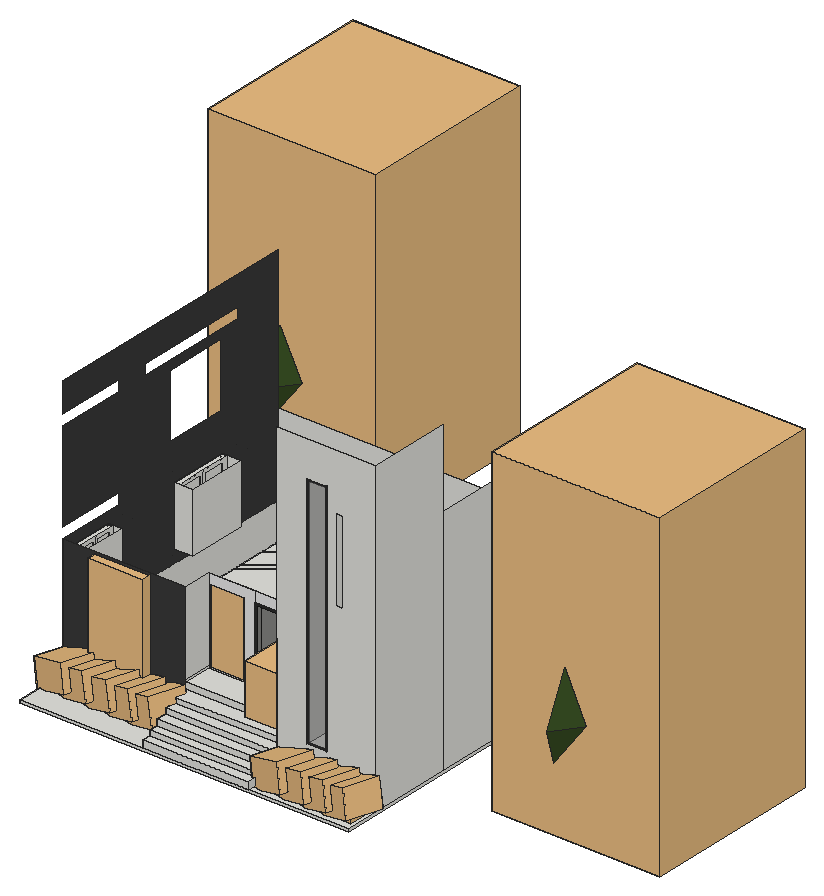
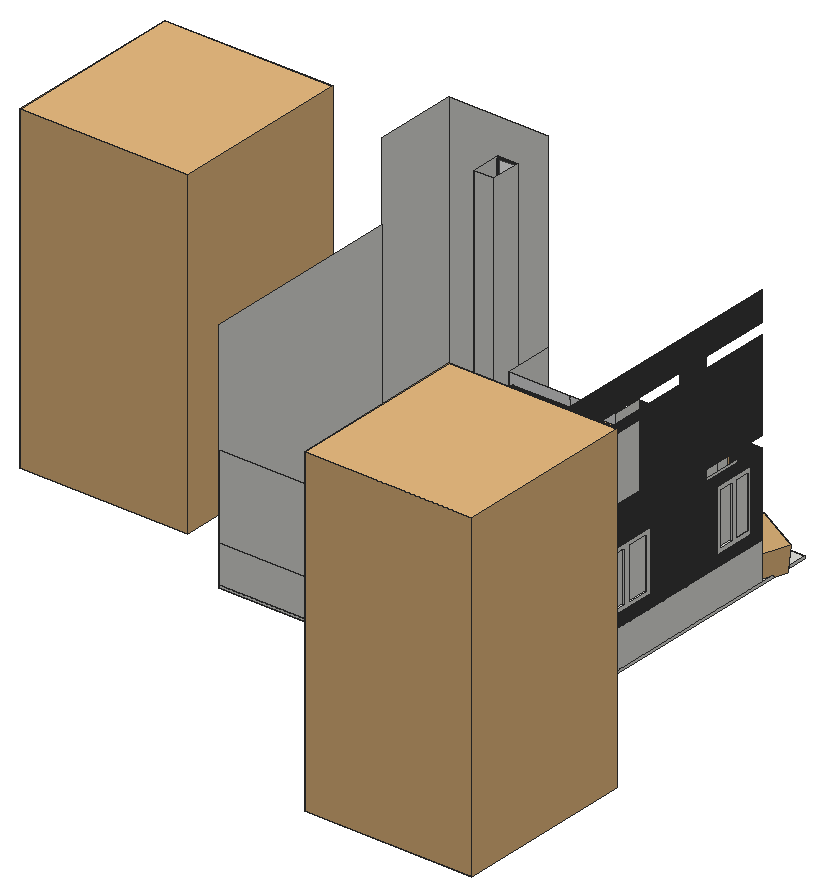
# SketchUp Ruby script. Lengths in inches.
U = 1.inch
M = Sketchup.active_model
def pt(a) = Geom::Point3d.new(a.map { |v| v * U })
def face(e, loops, mat)
  f = e.add_face(loops[0].map { |a| pt(a) })
  loops[1..].each { |l| e.add_face(l.map { |a| pt(a) }).erase! }
  f.material = f.back_material = mat if mat
  f
end
# faces: each face lists its corners as indices into pts; further lists are holes
def faces(e, pts, list, mat = nil) = list.each { |f| face(e, (f[0].is_a?(Array) ? f : [f]).map { |l| l.map { |i| pts[i] } }, mat) }
# xy, xz, yz: faces in a plane at the given z, y or x. An outline is a flat list of corners, or four numbers for a rectangle; further outlines are holes
def ring(l) = l.size == 4 ? [[l[0], l[1]], [l[2], l[1]], [l[2], l[3]], [l[0], l[3]]] : l.each_slice(2).to_a
def flat(e, list, mat, &to3) = list.each { |f| face(e, (f[0].is_a?(Array) ? f : [f]).map { |l| ring(l).map { |u, v| to3.(u, v) } }, mat) }
def xy(e, z, list, mat = nil) = flat(e, list, mat) { |x, y| [x, y, z] }
def xz(e, y, list, mat = nil) = flat(e, list, mat) { |x, z| [x, y, z] }
def yz(e, x, list, mat = nil) = flat(e, list, mat) { |y, z| [x, y, z] }
def lines(e, pts, list) = list.each { |a, b| e.add_line(pt(pts[a]), pt(pts[b])) }
# prism: a flat outline (further loops are holes) pulled along v
def prism(e, loops, v, mat = nil)
  f = face(e, loops, mat); d = Geom::Vector3d.new(v.map { |x| x * U })
  f.pushpull(f.normal.samedirection?(d) ? d.length : -d.length)
end
def box(e, o, s, mat = nil) = prism(e, [[o, [o[0] + s[0], o[1], o[2]], [o[0] + s[0], o[1] + s[1], o[2]], [o[0], o[1] + s[1], o[2]]]], [0, 0, s[2]], mat)
def at(x, y, z, deg = 0) = Geom::Transformation.translation(pt([x, y, z])) * Geom::Transformation.rotation(ORIGIN, Z_AXIS, deg.degrees)
def axes(o, x, y, z) = Geom::Transformation.new([*x, 0, *y, 0, *z, 0, *pt(o).to_a, 1])
def part(name) = M.definitions.add(name)
# library, detail: a bought-in or finely detailed component or shape, given as its bounding box
def library(name, o, s) = part(name).tap { |d| box(d.entities, o, s) }
def detail(e, o, s) = box(e.add_group.entities, o, s)
def put(e, d, t, mat = nil) = e.add_instance(d, t).tap { |i| i.material = mat if mat }
def group(e, t, mat = nil) = e.add_group.tap { |g| g.transformation = t; g.material = mat if mat }.entities
root = M.entities
M.materials.add("AM113_062_Tilia").color = [58, 81, 37]
M.materials.add("AM113_062_Tilia_Bark").color = [88, 85, 72]
M.materials.add("Glass_Tinted_Gray").color = [0, 0, 0]
M.materials["Glass_Tinted_Gray"].alpha = 0.125
M.materials.add("Material__1").color = [190, 136, 85]
M.materials.add("Material__2").color = [51, 42, 44]
M.materials.add("Material__3").color = [119, 136, 107]
M.materials.add("[0135_DarkGray]").color = [81, 81, 81]
M.materials.add("[Color M07]").color = [58, 58, 58]
M.materials.add("[Mirror 02]").color = [229, 229, 229]
M.materials.add("[Terrazzo Light Blue]").color = [196, 214, 227]
M.materials.add("[Translucent Glass Gray]1").color = [128, 128, 128]
M.materials["[Translucent Glass Gray]1"].alpha = 0.5
M.materials.add("white_wall").color = [233, 233, 233]
c1 = library("\#2",[-119.83,-119.83,113.8],[239.66,239.66,17.4])
c2 = library("\#4",[-204.92,-212.35,-236.71],[424.28,257.5,472.53])
c3 = part("\#3")
put(c3.entities,c2,axes([-0.37,309.72,0],[1.36765,0,0],[0,1.36765,0],[0,0,1.36765]),"Material__3")
c4 = library("\#1",[-174.07,-174.07,0],[348.14,348.14,140])
c5 = part("9")
put(c5.entities,c1,at(-19.94,-24.66,0),"Material__2")
put(c5.entities,c3,axes([17.67,-32.6,40.29],[0.29694,0.9549,0],[-0.21403,0.06656,0.97456],[0.9306,-0.28939,0.22414]))
put(c5.entities,c4,at(-19.94,-24.66,0),"Material__1")
c6 = library("AM113_062_Tilia_Defintion",[-350.67,-364.73,-2.58],[672.29,726.36,1000])
c7 = library("Shrub+_Grass",[-121.83,-22.34,0],[123.96,19.94,123.95])
c8 = library("Plant",[-21.8,-11.875,0],[94.69,106.42,111.78])
c9 = library("PINTU+6+YA",[0,-0.6875,0],[35.83,8.07,80.71])
c10 = part("PENTEK_RP Fineline 50S_Sliding_DoorCase_E1")
box(c10.entities,[0,0,0],[1.51,3.66,99.27],"[0135_DarkGray]")
c11 = part("PENTEK_RP Fineline 50S_SlidingDooe_Case_E2")
box(c11.entities,[0,0,0],[96.25,3.66,1.51],"[0135_DarkGray]")
c12 = part("pentek_RP Fineline 50S_SlidingDoor_Case")
put(c12.entities,c10,at(97.76,0,0))
put(c12.entities,c11,at(1.51,0,0))
put(c12.entities,c10,at(0,0,0))
put(c12.entities,c11,at(1.51,0,97.76))
c13 = part("PENTEK_RP Fineline 50S_SlidingDoor_GlazingBead_2")
box(c13.entities,[0,0,0],[0.56,0.59,94.39],"[0135_DarkGray]")
c14 = part("PENTEK_RP Fineline 50S_SlidingDoor_Glass")
box(c14.entities,[0,0,0],[46.58,0.16,94.39],"Glass_Tinted_Gray")
c15 = part("PENTEK_RP Fineline 50S_SlidingDoor_GlazingBead")
box(c15.entities,[0,0,0],[45.47,0.59,0.56],"[0135_DarkGray]")
c16 = part("PENTEK_RP Fineline 50S_SlidingDoor_Leaf_E1")
xy(c16.entities,0,[[0,0,0.93,1.97],[0.93,1.57,1.49,1.97]],"[0135_DarkGray]")
xy(c16.entities,96.25,[[0,0,0.93,0,0.93,1.57,1.49,1.57,1.49,1.97,0,1.97]],"[0135_DarkGray]")
xz(c16.entities,0,[[0,0,0.93,96.25]],"[0135_DarkGray]")
xz(c16.entities,1.57,[[0.93,0,1.49,95.32],[0.93,95.32,1.49,96.25]],"[0135_DarkGray]")
xz(c16.entities,1.97,[[0,0,1.49,96.25]],"[0135_DarkGray]")
yz(c16.entities,0,[[0,0,1.97,96.25]],"[0135_DarkGray]")
yz(c16.entities,0.93,[[0,0,1.57,0.93],[0,0.93,1.57,95.32],[0,95.32,1.57,96.25]],"[0135_DarkGray]")
yz(c16.entities,1.49,[[1.57,0,1.97,95.32],[1.57,95.32,1.97,96.25]],"[0135_DarkGray]")
c17 = part("PENTEK_RP Fineline 50S_SlidingDoor_Leaf_E2")
xy(c17.entities,0,[[0,0,0,1.57,0.56,1.57,0.56,1.97,46.02,1.97,46.02,1.57,46.58,1.57,46.58,0]],"[0135_DarkGray]")
xy(c17.entities,0.93,[[0,0,46.58,1.57]],"[0135_DarkGray]")
xy(c17.entities,1.49,[[0.56,1.57,46.02,1.97]],"[0135_DarkGray]")
xz(c17.entities,0,[[0,0,46.58,0.93]],"[0135_DarkGray]")
xz(c17.entities,1.57,[[0,0,0.56,0.93],[46.02,0,46.58,0.93],[0.56,0.93,46.02,1.49]],"[0135_DarkGray]")
xz(c17.entities,1.97,[[0.56,0,46.02,1.49]],"[0135_DarkGray]")
yz(c17.entities,0,[[0,0,1.57,0.93]],"[0135_DarkGray]")
yz(c17.entities,0.56,[[1.57,0,1.97,0.93],[1.57,0.93,1.97,1.49]],"[0135_DarkGray]")
yz(c17.entities,46.02,[[1.57,0,1.97,0.93],[1.57,0.93,1.97,1.49]],"[0135_DarkGray]")
yz(c17.entities,46.58,[[0,0,1.57,0.93]],"[0135_DarkGray]")
c18 = part("PENTEK_RP Fineline S_SlidingDoor_Leaf1")
put(c18.entities,c13,at(0.93,0,0.93))
put(c18.entities,c13,at(46.96,0,0.93))
put(c18.entities,c14,at(1.49,1.42,0.93))
put(c18.entities,c15,at(1.49,0,0.93))
put(c18.entities,c14,at(1.49,0.59,0.93),"[Terrazzo Light Blue]")
put(c18.entities,c16,at(0,0,0))
put(c18.entities,c16,axes([48.44,0,0],[-1,0,0],[0,1,0],[0,0,1]))
put(c18.entities,c17,axes([0.93,0,96.25],[1,0,0],[0,1,0],[0,0,-1]))
put(c18.entities,c17,at(0.93,0,0))
put(c18.entities,c15,at(1.49,0,94.77))
c19 = part("PENTEK_RP Fineline 50S_SlidingDoor_Leaf2")
put(c19.entities,c14,at(1.49,1.42,0.93))
put(c19.entities,c15,at(1.49,0,94.77))
put(c19.entities,c13,at(46.96,0,0.93))
put(c19.entities,c14,at(1.49,0.59,0.93),"[Mirror 02]")
put(c19.entities,c13,at(0.93,0,0.93))
put(c19.entities,c16,at(0,0,0))
put(c19.entities,c16,axes([48.44,0,0],[-1,0,0],[0,1,0],[0,0,1]))
put(c19.entities,c15,at(1.49,0,0.93))
put(c19.entities,c17,axes([0.93,0,96.25],[1,0,0],[0,1,0],[0,0,-1]))
put(c19.entities,c17,at(0.93,0,0))
c20 = part("PENTEK - Slimmest Steel Sliding Door / Window\#1")
put(c20.entities,c12,at(0,-1.88,-0.09))
put(c20.entities,c18,at(1.51,-2.27,1.42))
put(c20.entities,c19,at(49.32,-0.3,1.42))
c21 = part("Window (2)")
xy(c21.entities,31.72,[[-0.78,88.6,2.72,128.1]])
xy(c21.entities,34.95,[[-0.78,91.53,0.84,106.59],[0.84,91.53,1.05,97.58],[1.05,91.53,1.42,106.59],[1.42,91.53,2.72,106.59],[0.84,97.58,1.05,98.18],
  [0.84,98.18,1.05,106.59]])
xy(c21.entities,35.27,[[-0.78,110.09,0.97,125.14],[1.05,110.09,2.72,125.14]])
xy(c21.entities,58.35,[[2.72,108.74,3.8,109.74]])
xy(c21.entities,77.8125,[[-0.78,110.09,2.72,125.14],[0.97,110.09,1.05,125.14]])
xy(c21.entities,77.93,[[-0.78,91.53,0.84,106.59],[1.05,91.53,1.42,106.59],[1.42,91.53,2.72,106.59]])
xy(c21.entities,80.72,[[-0.78,88.6,2.72,128.1]])
xz(c21.entities,88.6,[[-0.78,31.72,2.72,80.72]])
xz(c21.entities,91.53,[[-0.78,34.95,0.84,77.93],[1.05,34.95,1.42,77.93],[1.42,34.95,2.72,77.93]])
xz(c21.entities,106.59,[[-0.78,34.95,0.84,77.93],[0.84,34.95,1.05,77.93],[0.84,34.95,2.72,77.93]])
xz(c21.entities,108.74,[[3.8,54.35,4.22,54.6,4.22,59.47,2.72,59.97,2.72,58.35,3.8,58.35]])
xz(c21.entities,109.74,[[3.8,54.35,3.8,58.35,2.72,58.35,2.72,59.97,4.22,59.47,4.22,54.6]])
xz(c21.entities,110.09,[[-0.78,35.27,0.97,77.8125],[1.05,35.27,2.72,77.8125]])
xz(c21.entities,125.14,[[-0.78,35.27,0.97,77.8125],[0.97,35.27,1.05,80.72],[1.05,35.27,2.72,77.8125]])
xz(c21.entities,128.1,[[-0.78,31.72,2.72,80.72]])
yz(c21.entities,-0.78,[[[88.6,31.72,128.1,80.72],[91.53,34.95,106.59,77.93],[110.09,35.27,125.14,77.8125]]])
yz(c21.entities,0.84,[[91.53,34.95,106.59,77.93]])
yz(c21.entities,0.97,[[110.09,35.27,125.14,77.8125]])
yz(c21.entities,1.05,[[91.53,34.95,106.59,77.93],[110.09,35.27,125.14,77.8125]])
yz(c21.entities,1.42,[[91.53,34.95,106.59,77.93]])
yz(c21.entities,2.72,[[[88.6,31.72,108.35,80.72],[91.53,34.95,106.59,77.93]],[[108.35,31.72,128.1,80.72],[110.09,35.27,125.14,77.8125],[108.74,58.35,109.74,59.97]]])
yz(c21.entities,3.8,[[108.74,54.35,109.74,58.35]])
yz(c21.entities,4.22,[[108.74,54.6,109.74,59.47]])
p = [[4.22,108.74,54.6],[3.8,108.74,54.35],[3.8,109.74,54.35],[4.22,109.74,54.6],[2.72,109.74,59.97],[2.72,108.74,59.97],
  [4.22,108.74,59.47],[4.22,109.74,59.47],[-0.78,86.4,89.94],[-0.78,86.44,89.94],[15.22,130.69,89.94],[15.22,130.65,89.94],
  [-0.78,86.44,28.19],[-0.78,86.4,28.19],[7.72,130.69,89.94],[7.72,130.65,89.94]]
faces(c21.entities,p,[[0,1,2,3],[4,5,6,7]])
lines(c21.entities,p,[[8,9],[10,11],[12,13],[14,15]])
xy(root,1.25,[[695.48,0,695.48,121.6875,418.81,121.6875,418.81,725.65,1160.625,725.65,1160.625,76.875,935.92,76.875,935.92,0]])
xy(root,17.91,[[695.48,0,935.92,19.6875]])
xy(root,28.84,[[695.48,19.6875,935.92,40.375]])
xy(root,42.15,[[695.48,40.375,935.92,64.0625]])
xy(root,54.11,[[695.48,64.0625,935.92,89.1875]])
xy(root,66.27,[[695.48,89.1875,935.92,121.6875]])
xy(root,80.94,[[695.48,121.6875,935.92,187.1875]])
xy(root,84,[[1005.08,76.875,1049.99,143.25]])
xy(root,84.75,[[699,187.1875,773.61,220.1875]])
xy(root,94.03,[[798.31,187.1875,927.68,205.0625]])
xy(root,105.22,[[496.21,121.6875,613.65,148.5625]])
xy(root,109.98,[[418.81,151.95,449.99,247.52]])
xy(root,115.22,[[418.81,435.18,460.62,569.75]])
xz(root,0,[[695.48,1.25,935.92,17.91]])
xz(root,19.6875,[[695.48,17.91,935.92,28.84]])
xz(root,40.375,[[695.48,28.84,935.92,42.15]])
xz(root,64.0625,[[695.48,42.15,935.92,54.11]])
xz(root,76.875,[[[935.92,1.25,1160.625,701.22],[1005.08,84,1049.99,620.81],[1069.1,385.18,1085.03,573.56]]])
xz(root,89.1875,[[695.48,54.11,935.92,66.27]])
xz(root,121.6875,[[695.48,66.27,935.92,80.94]])
xz(root,121.6875,[[[418.81,1.25,695.48,273.04],[496.21,105.22,613.65,249.78]]],"[Color M07]")
xz(root,143.25,[[1005.08,84,1049.99,620.81]])
xz(root,148.5625,[[496.21,105.22,613.65,249.78]])
xz(root,151.95,[[418.81,109.98,449.99,249.78]])
xz(root,187.1875,[[695.48,80.94,935.92,84.75]])
xz(root,187.1875,[[695.48,84.75,699,84.75,699,249.78,773.61,249.78,773.61,84.75,798.31,84.75,798.31,273.04,695.48,273.04],[798.31,84.75,935.92,84.75,935.92,273.04,798.31,273.04,798.31,249.78,927.68,249.78,927.68,94.03,798.31,94.03]],"white_wall")
xz(root,205.0625,[[798.31,94.03,927.68,249.78]])
xz(root,220.1875,[[699,84.75,773.61,249.78]])
xz(root,247.52,[[418.81,109.98,449.99,249.78]])
xz(root,435.18,[[418.81,115.22,460.62,249.78]])
xz(root,569.75,[[418.81,115.22,460.62,249.78]])
xz(root,725.65,[[418.81,1.25,1160.625,84.75],[418.81,84.75,1160.625,273.04]])
yz(root,418.81,[[121.6875,1.25,725.65,84.75]])
yz(root,418.81,[[[121.6875,84.75,121.6875,273.04,278.26,273.04,278.26,297.35,121.6875,297.35,121.6875,500.91,278.26,500.91,278.26,525.1,121.6875,525.1,121.6875,592.47,725.65,592.47,725.65,84.75],[422.72,336.96,567.03,481.27],[435.18,115.22,569.75,249.78],[151.95,109.98,247.52,249.78],[353.16,500.91,615.47,525.1]]],"[Color M07]")
yz(root,449.99,[[151.95,109.98,247.52,249.78]])
yz(root,460.62,[[435.18,115.22,569.75,249.78]])
yz(root,496.21,[[121.6875,105.22,148.5625,249.78]])
yz(root,613.65,[[121.6875,105.22,148.5625,249.78]])
yz(root,695.48,[[0,1.25,0,17.91,19.6875,17.91,19.6875,28.84,40.375,28.84,40.375,42.15,64.0625,42.15,64.0625,54.11,89.1875,54.11,89.1875,66.27,121.6875,66.27,121.6875,1.25],[121.6875,80.94,187.1875,84.75],[121.6875,84.75,187.1875,273.04]])
yz(root,699,[[187.1875,84.75,220.1875,249.78]])
yz(root,773.61,[[187.1875,84.75,220.1875,249.78]])
yz(root,798.31,[[187.1875,94.03,205.0625,249.78]])
yz(root,927.68,[[187.1875,94.03,205.0625,249.78]])
yz(root,935.92,[[0,1.25,76.875,1.25,76.875,54.11,64.0625,54.11,64.0625,42.15,40.375,42.15,40.375,28.84,19.6875,28.84,19.6875,17.91,0,17.91],[76.875,54.11,76.875,84.75,187.1875,84.75,187.1875,80.94,121.6875,80.94,121.6875,66.27,89.1875,66.27,89.1875,54.11],[76.875,84.75,187.1875,273.04]])
yz(root,1005.08,[[76.875,84,143.25,620.81]])
yz(root,1049.99,[[76.875,84,143.25,620.81]])
yz(root,1160.625,[[76.875,1.25,265.5,701.22],[265.5,1.25,725.65,525.1]])
p = [[1526.7,99.61,282.39],[1507.42,143.31,193.84],[1537.24,198.77,252.375],[366.07,748.39,282.39],[346.79,792.08,193.84],[376.62,847.54,252.375],
  [1490.22,196.7,355.05],[329.59,845.48,355.05]]
faces(root,p,[[0,1,2],[3,4,5],[0,2,6],[3,5,7]],"AM113_062_Tilia")
put(root,c5,axes([1130.03,43.88,-2.35],[0.1342,0,0],[0,0.1342,0],[0,0,0.17849]))
put(root,c5,axes([1035.59,43.88,-2.35],[0.1342,0,0],[0,0.1342,0],[0,0,0.17849]))
put(root,c5,axes([981.28,43.88,-2.35],[0.1342,0,0],[0,0.1342,0],[0,0,0.17849]))
put(root,c5,axes([1084.78,43.88,-2.35],[0.1342,0,0],[0,0.1342,0],[0,0,0.17849]))
g1 = group(root,at(418.14,40.73,-2.35))
put(g1,c5,axes([239.2,45.89,0],[0.1342,0,0],[0,0.1342,0],[0,0,0.17849]))
put(g1,c5,axes([144.76,45.89,0],[0.1342,0,0],[0,0.1342,0],[0,0,0.17849]))
put(g1,c5,axes([90.45,45.89,0],[0.1342,0,0],[0,0.1342,0],[0,0,0.17849]))
put(g1,c5,axes([193.95,45.89,0],[0.1342,0,0],[0,0.1342,0],[0,0,0.17849]))
put(g1,c5,axes([42.2,45.89,0],[0.1342,0,0],[0,0.1342,0],[0,0,0.17849]))
g2 = group(root,at(418.81,725.65,-36.1875))
box(g2,[0,-725.65,31.4375],[741.82,725.65,6])
put(root,c6,axes([353.72,1062.62,3.12],[0.56218,0,0],[0,0.56218,0],[0,0,0.72521]),"AM113_062_Tilia_Bark")
put(root,c6,axes([1514.34,413.85,3.12],[0.56218,0,0],[0,0.56218,0],[0,0,0.72521]),"AM113_062_Tilia_Bark")
put(root,c7,axes([612.24,125,43],[1,0,0],[0,1,0],[0,0,1.815]))
put(root,c8,at(874.97,101.8125,80.94))
g3 = group(root,at(1005.08,76.875,84))
xy(g3,0,[[0,0,44.9,1.875]],"[Color M07]")
xy(g3,3.09,[[3.09,0,41.81,1.875]],"[Color M07]")
xy(g3,533.72,[[3.09,0,41.81,1.875]],"[Color M07]")
xy(g3,536.8125,[[0,0,44.9,1.875]],"[Color M07]")
xz(g3,0,[[[0,0,44.9,536.8125],[3.09,3.09,41.81,533.72]]],"[Color M07]")
xz(g3,0,[[3.09,3.09,41.81,533.72]],"[Translucent Glass Gray]1")
xz(g3,1.875,[[[0,0,44.9,536.8125],[3.09,3.09,41.81,533.72]]],"[Color M07]")
yz(g3,0,[[0,0,1.875,536.8125]],"[Color M07]")
yz(g3,3.09,[[0,3.09,1.875,533.72]],"[Color M07]")
yz(g3,41.81,[[0,3.09,1.875,533.72]],"[Color M07]")
yz(g3,44.9,[[0,0,1.875,536.8125]],"[Color M07]")
put(root,c9,axes([699,187.1875,84.75],[2.08229,0,0],[0,1,0],[0,0,2.04476]))
put(root,c20,axes([798.31,189.33,94.17],[1.30323,0,0],[0,1,0],[0,0,1.56892]))
put(root,c21,axes([421.25,-67.59,21.94],[3.1248,0,0],[0,2.46154,0],[0,0,2.80496]))
put(root,c20,axes([496.21,123.56,105.35],[1.18298,0,0],[0,1,0],[0,0,1.45622]))
put(root,c21,axes([421.25,136.98,29.29],[3.1248,0,0],[0,3.37197,0],[0,0,2.72326]))
